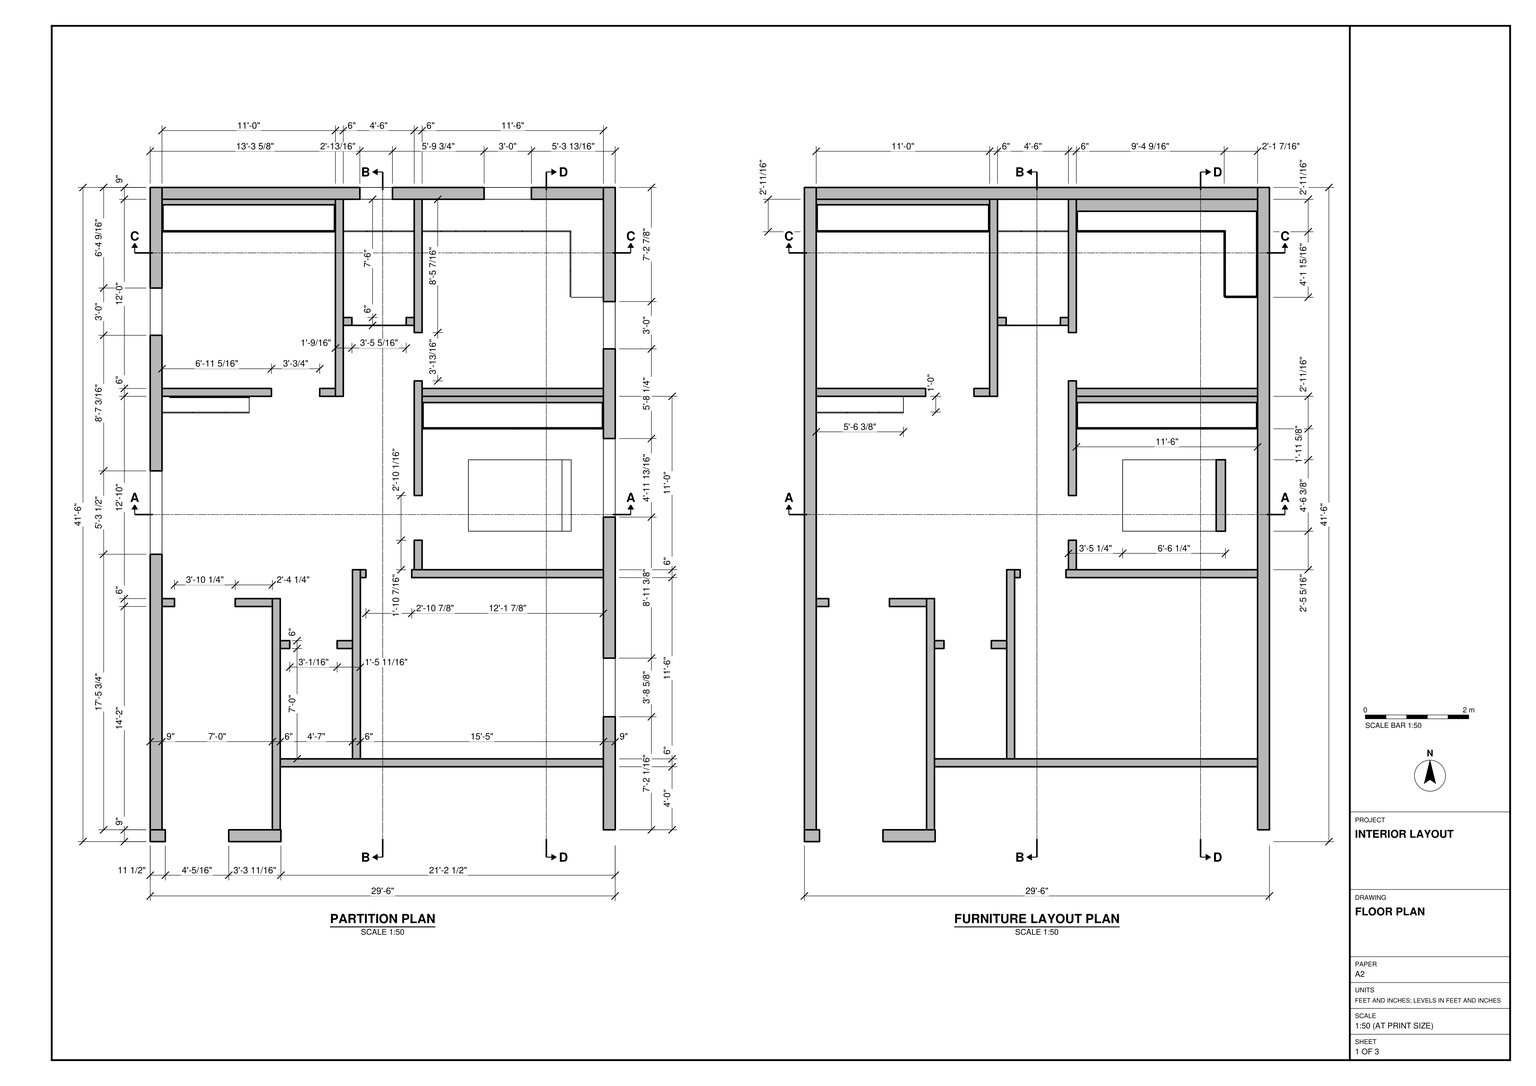
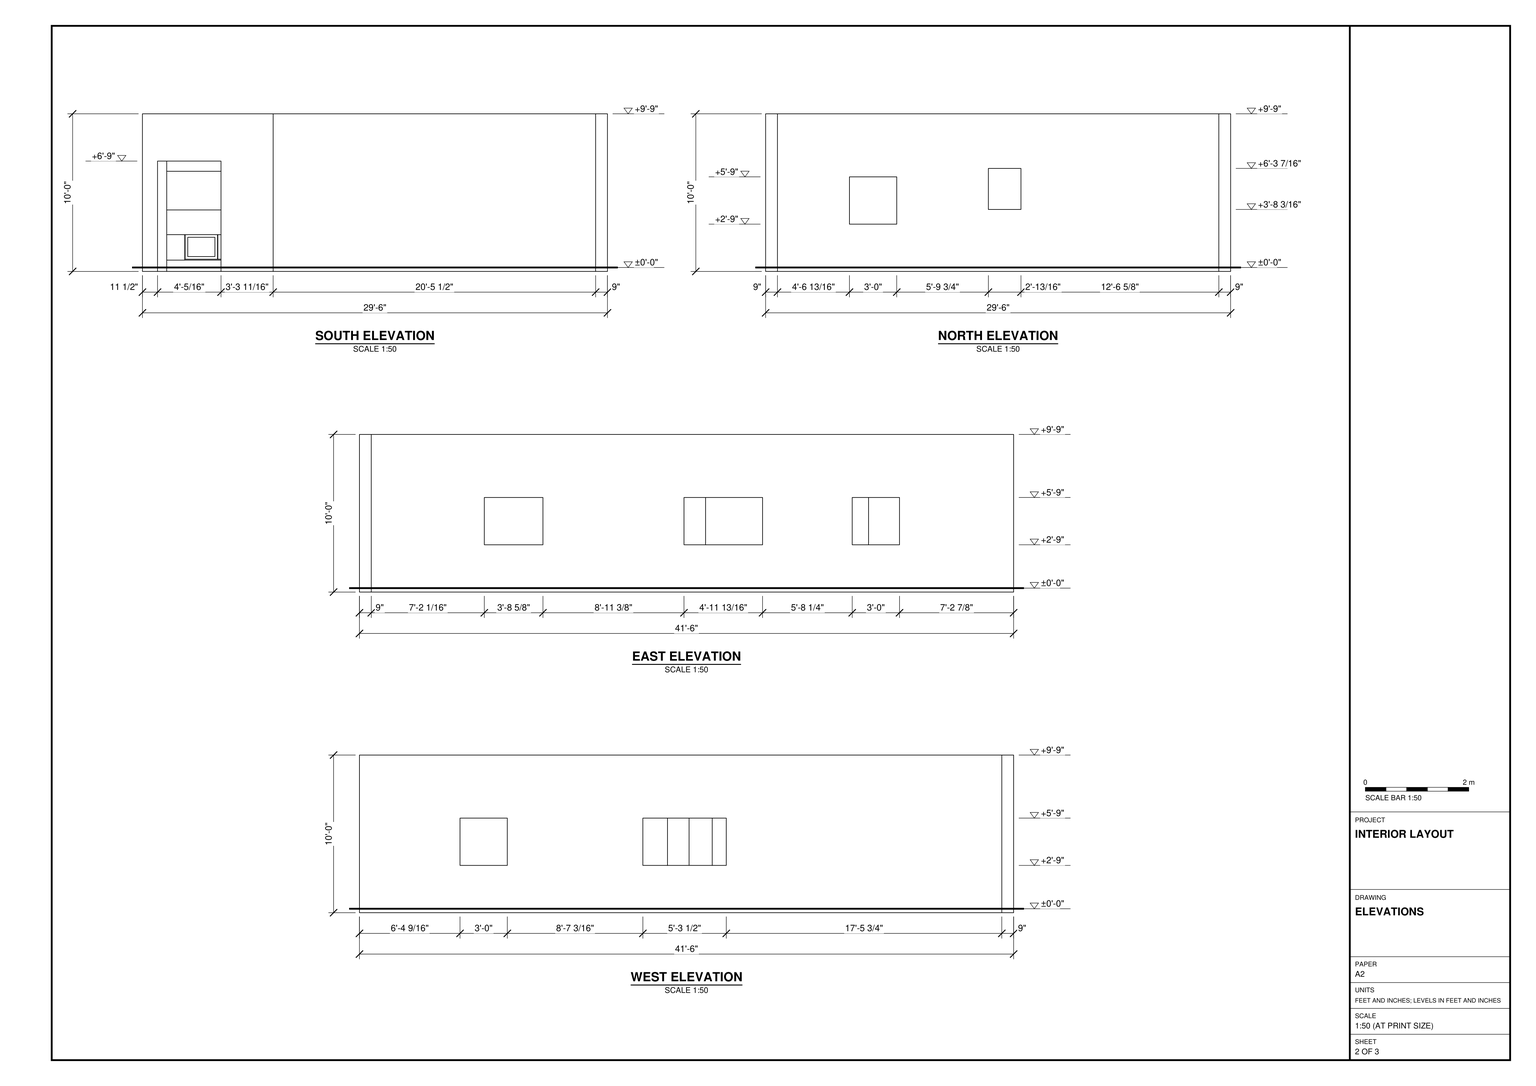
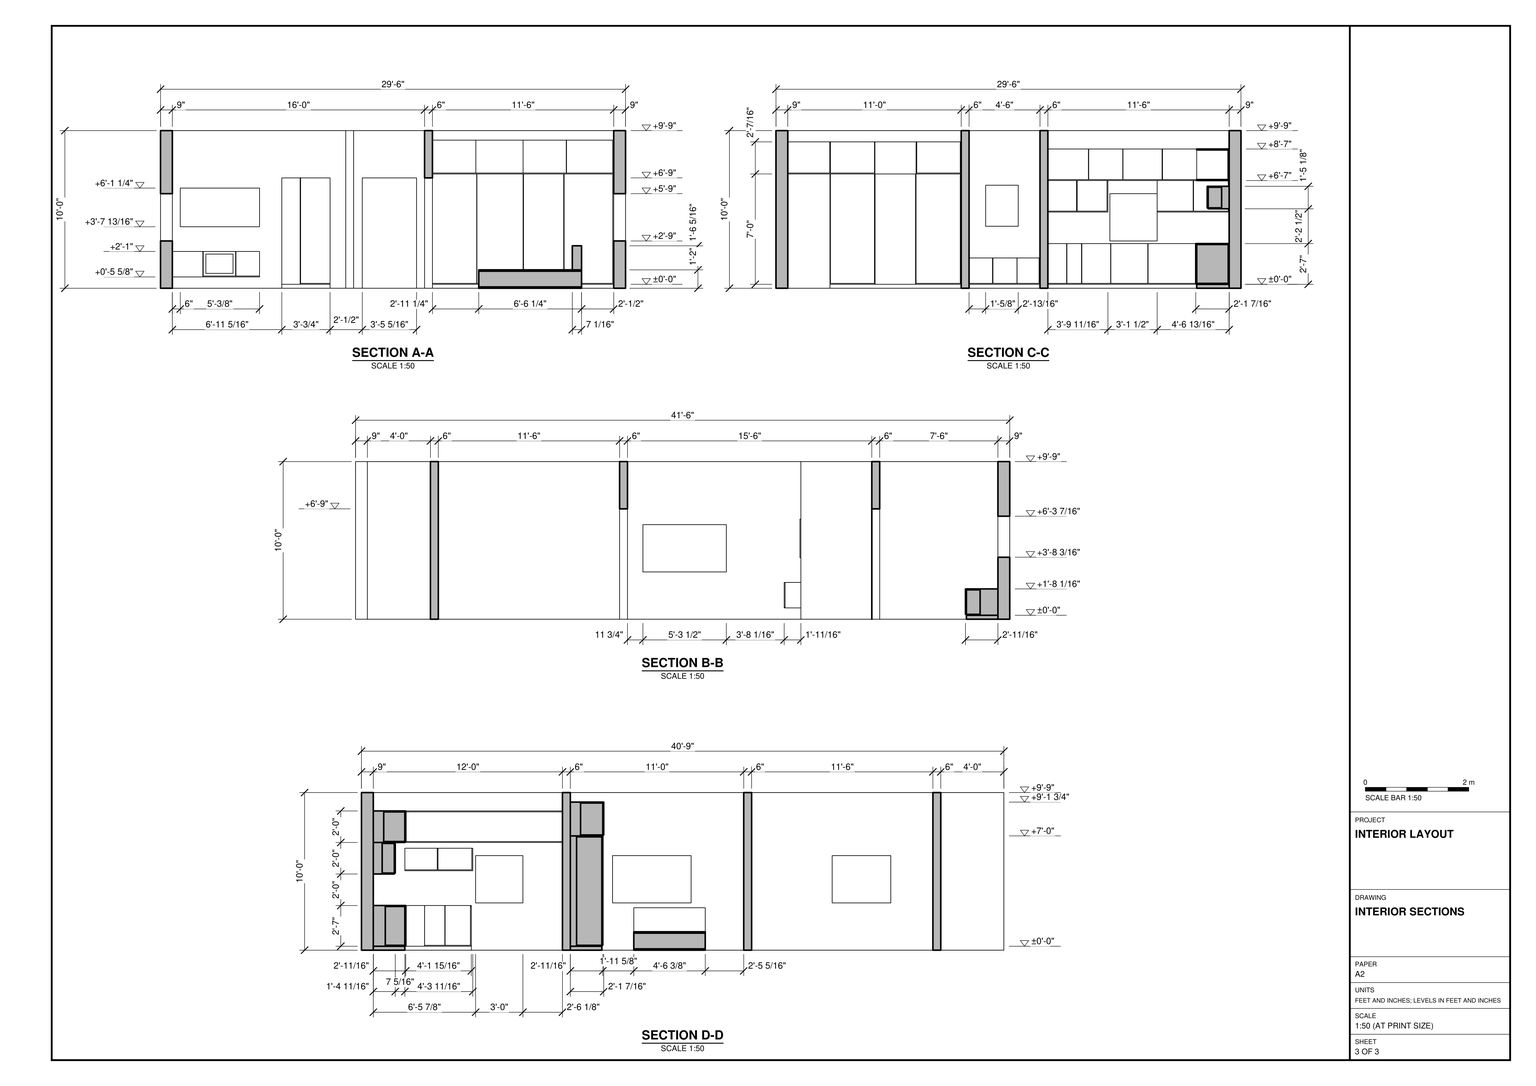
Build the interior in SketchUp from task_files/diagram_01.pdf. Work in feet and inches. Set the ground floor at ±0'-0" and make the model 29'-6" wide east to west, 41'-6" long north to south and 10'-0" high overall. The wall tops are at +9'-9" relative to the floor.

Use the partition plan to lay out the 9" perimeter walls and 6" internal partitions. Follow the setback at the south end, the narrow southwest entrance bay, the passages between rooms and the narrow bay between the two north rooms. Use the elevations to set the widths, sills and heads of the exterior openings; the two north windows have different sill heights.

Use the furniture plan for footprints and the interior sections for heights and cabinet divisions. Model the northwest storage run, the northeast kitchen cabinetry and its return, and the low wall unit on the passage side of the northwest room. Place the platform bed in the middle east room with its raised end to the east and the storage run along the north partition. Any decor or loose items shown may be represented by suitable library components.

Keep shell elements separate as groups or components, group each furniture or joinery piece separately, and use components for repeated parts. Save one SketchUp model as output_files/interior_with_fitted_cabinetry_and_platform_bed.skp.

# SketchUp Ruby script. Lengths in inches.
U = 1.inch
M = Sketchup.active_model
def pt(a) = Geom::Point3d.new(a.map { |v| v * U })
def face(e, loops, mat)
  f = e.add_face(loops[0].map { |a| pt(a) })
  loops[1..].each { |l| e.add_face(l.map { |a| pt(a) }).erase! }
  f.material = f.back_material = mat if mat
  f
end
# faces: each face lists its corners as indices into pts; further lists are holes
def faces(e, pts, list, mat = nil) = list.each { |f| face(e, (f[0].is_a?(Array) ? f : [f]).map { |l| l.map { |i| pts[i] } }, mat) }
# xy, xz, yz: faces in a plane at the given z, y or x. An outline is a flat list of corners, or four numbers for a rectangle; further outlines are holes
def ring(l) = l.size == 4 ? [[l[0], l[1]], [l[2], l[1]], [l[2], l[3]], [l[0], l[3]]] : l.each_slice(2).to_a
def flat(e, list, mat, &to3) = list.each { |f| face(e, (f[0].is_a?(Array) ? f : [f]).map { |l| ring(l).map { |u, v| to3.(u, v) } }, mat) }
def xy(e, z, list, mat = nil) = flat(e, list, mat) { |x, y| [x, y, z] }
def xz(e, y, list, mat = nil) = flat(e, list, mat) { |x, z| [x, y, z] }
def yz(e, x, list, mat = nil) = flat(e, list, mat) { |y, z| [x, y, z] }
def lines(e, pts, list) = list.each { |a, b| e.add_line(pt(pts[a]), pt(pts[b])) }
# prism: a flat outline (further loops are holes) pulled along v
def prism(e, loops, v, mat = nil)
  f = face(e, loops, mat); d = Geom::Vector3d.new(v.map { |x| x * U })
  f.pushpull(f.normal.samedirection?(d) ? d.length : -d.length)
end
def box(e, o, s, mat = nil) = prism(e, [[o, [o[0] + s[0], o[1], o[2]], [o[0] + s[0], o[1] + s[1], o[2]], [o[0], o[1] + s[1], o[2]]]], [0, 0, s[2]], mat)
def at(x, y, z, deg = 0) = Geom::Transformation.translation(pt([x, y, z])) * Geom::Transformation.rotation(ORIGIN, Z_AXIS, deg.degrees)
def axes(o, x, y, z) = Geom::Transformation.new([*x, 0, *y, 0, *z, 0, *pt(o).to_a, 1])
def part(name) = M.definitions.add(name)
# library, detail: a bought-in or finely detailed component or shape, given as its bounding box
def library(name, o, s) = part(name).tap { |d| box(d.entities, o, s) }
def detail(e, o, s) = box(e.add_group.entities, o, s)
def put(e, d, t, mat = nil) = e.add_instance(d, t).tap { |i| i.material = mat if mat }
def group(e, t, mat = nil) = e.add_group.tap { |g| g.transformation = t; g.material = mat if mat }.entities
root = M.entities
M.materials.add("[Translucent Glass Safety]").color = [204, 235, 244]
M.materials["[Translucent Glass Safety]"].alpha = 0.5
xz(root,393,[[153.57,0,194.89,84]],"[Translucent Glass Safety]")
g1 = group(root,at(0,0,0))
prism(g1,[[[99.51,9,0],[59.8125,9,0],[59.8125,9,84],[11.5,9,84],[11.5,9,0],[0,9,0],[0,9,120],[99.51,9,120]]],[0,-9,0])
g2 = group(root,at(0,9,0))
prism(g2,[[[0,489,0],[0,0,0],[0,0,120],[0,489,120]],[[0,273.25,72],[0,209.75,72],[0,209.75,36],[0,273.25,36]],[[0,412.4375,72],[0,376.4375,72],[0,376.4375,36],[0,412.4375,36]]],[9,0,0])
g3 = group(root,at(9,489,0))
prism(g3,[[[336,9,0],[0,9,0],[0,9,120],[336,9,120]],[[245.1875,9,36],[281.1875,9,36],[281.1875,9,72],[245.1875,9,72]],[[150.625,9,47.1875],[175.4375,9,47.1875],[175.4375,9,78.4375],[150.625,9,78.4375]]],[0,-9,0])
g4 = group(root,at(345,9,0))
prism(g4,[[[9,0,0],[9,489,0],[9,489,120],[9,0,120]],[[9,297.875,36],[9,238.0625,36],[9,238.0625,72],[9,297.875,72]],[[9,130.6875,36],[9,86.0625,36],[9,86.0625,72],[9,130.6875,72]],[[9,366.125,36],[9,366.125,72],[9,402.125,72],[9,402.125,36]]],[-9,0,0])
g5 = group(root,at(9,179,0))
prism(g5,[[[9.5,6,0],[0,6,0],[0,6,120],[84,6,120],[84,6,0],[55.73,6,0],[55.73,6,84],[9.5,6,84]]],[0,-6,0])
g6 = group(root,at(93,9,0))
box(g6,[0,0,0],[6,176,120])
g7 = group(root,at(99,57,0))
box(g7,[0,0,0],[246,6,120])
g8 = group(root,at(154,63,0))
box(g8,[0,0,0],[6,144,120])
g9 = group(root,at(99,147,0))
prism(g9,[[[55,6,0],[43.3125,6,0],[43.3125,6,84],[7.25,6,84],[7.25,6,0],[0,6,0],[0,6,120],[55,6,120]]],[0,-6,0])
g10 = group(root,at(160,201,0))
prism(g10,[[[4.25,6,0],[0,6,0],[0,6,120],[185,6,120],[185,6,0],[39.125,6,0],[39.125,6,84],[4.25,6,84]]],[0,-6,0])
g11 = group(root,at(141,339,0))
prism(g11,[[[6,0,0],[0,0,0],[0,6,0],[0,150,0],[6,150,0]]],[0,0,120])
g12 = group(root,at(9,339,0))
prism(g12,[[[0,0,0],[83.3125,0,0],[83.3125,0,84],[120.0625,0,84],[120.0625,0,0],[132,0,0],[132,0,120],[0,0,120]]],[0,6,0])
g13 = group(root,at(147,393,0))
prism(g13,[[[6.57,6,0],[0,6,0],[0,6,120],[54,6,120],[54,6,0],[47.89,6,0],[47.89,6,84],[6.57,6,84]]],[0,-6,0])
g14 = group(root,at(201,207,0))
prism(g14,[[[0,282,0],[0,180.5625,0],[0,180.5625,84],[0,143.75,84],[0,143.75,0],[0,56.5,0],[0,56.5,84],[0,22.4375,84],[0,22.4375,0],[0,0,0],[0,0,120],[0,282,120]]],[6,0,0])
g15 = group(root,at(207,339,0))
box(g15,[0,0,0],[138,6,120])
g16 = group(root,at(207,465,0))
prism(g16,[[[0,0,0],[0,24,0],[138,24,0],[138,-50.625,0],[113.29,-50.625,0],[113.29,0,0]]],[0,0,3])
g17 = group(root,at(207,465,3))
xy(g17,0,[[113.29,-50.625,113.29,0,0,0,0,24,138,24,138,-50.625]])
xy(g17,0.71,[[113.29,-50.625,137.29,-50.625,137.29,14.875,0.71,14.875,0.71,0,113.29,0]])
xy(g17,30.29,[[113.29,-50.625,113.29,0,0.71,0,0.71,14.875,137.29,14.875,137.29,-50.625]])
xy(g17,31,[[113.29,-50.625,138,-50.625,138,24,0,24,0,0,113.29,0]])
xz(g17,-50.625,[[113.29,0,138,0,138,31,113.29,31,113.29,30.29,137.29,30.29,137.29,0.71,113.29,0.71]])
xz(g17,0,[[0,0,113.29,0,113.29,0.71,0.71,0.71,0.71,30.29,113.29,30.29,113.29,31,0,31]])
xz(g17,14.875,[[0.71,0.71,137.29,30.29]])
xz(g17,24,[[0,0,138,31]])
yz(g17,0,[[0,0,24,31]])
yz(g17,0.71,[[0,0.71,14.875,30.29]])
yz(g17,113.29,[[-50.625,0,0,0.71],[-50.625,30.29,0,31]])
yz(g17,137.29,[[-50.625,0.71,14.875,30.29]])
yz(g17,138,[[-50.625,0,24,31]])
g18 = group(root,at(320.29,414.375,3.71))
box(g18,[0,0,0],[24,0.71,29.58])
g19 = group(root,at(207,464.29,3.71))
box(g19,[0,0,0],[14.27,0.71,30.29])
g20 = group(root,at(221.48,464.29,3.71))
box(g20,[0,0,0],[11.13,0.71,30.29])
g21 = group(root,at(232.86,464.29,3.71))
box(g21,[0,0,0],[21.9,0.71,30.29])
g22 = group(root,at(254.93,464.29,3.71))
box(g22,[0,0,0],[28.12,0.71,30.29])
g23 = group(root,at(283.27,464.29,3.71))
box(g23,[0,0,0],[37.02,0.71,30.29])
g24 = group(root,at(319.58,449.99,3))
box(g24,[0,0,0],[0.71,13.97,31])
g25 = group(root,at(319.58,434.56,3.71))
box(g25,[0,0,0],[0.71,15.375,30.29])
g26 = group(root,at(319.58,415.08,3.71))
box(g26,[0,0,0],[0.71,19.26,30.29])
g27 = group(root,at(207,489,58))
xy(g27,0,[[0,-16,45.6875,0]])
xy(g27,0.71,[[0.71,-16,44.98,-5.75]])
xy(g27,23.29,[[0.71,-16,44.98,-5.75]])
xy(g27,24,[[0,-16,45.6875,0]])
xz(g27,-16,[[[0,0,45.6875,24],[0.71,0.71,44.98,23.29]]])
xz(g27,-5.75,[[0.71,0.71,44.98,23.29]])
xz(g27,0,[[0,0,45.6875,24]])
yz(g27,0,[[-16,0,0,24]])
yz(g27,0.71,[[-16,0.71,-5.75,23.29]])
yz(g27,44.98,[[-16,0.71,-5.75,23.29]])
yz(g27,45.6875,[[-16,0,0,24]])
g28 = group(root,at(207,472.29,58.71))
box(g28,[0,0,0],[21.81,0.71,23.29])
g29 = group(root,at(229.3125,472.29,58.71))
box(g29,[0,0,0],[22.66,0.71,23.29])
g30 = group(root,at(290.1875,489,58))
xy(g30,0,[[0,-16,54.8125,0]])
xy(g30,0.71,[[0.71,-16,54.1,-6.75]])
xy(g30,23.29,[[0.71,-16,54.1,-6.75]])
xy(g30,24,[[0,-16,54.8125,0]])
xz(g30,-16,[[[0,0,54.8125,24],[0.71,0.71,54.1,23.29]]])
xz(g30,-6.75,[[0.71,0.71,54.1,23.29]])
xz(g30,0,[[0,0,54.8125,24]])
yz(g30,0,[[-16,0,0,24]])
yz(g30,0.71,[[-16,0.71,-6.75,23.29]])
yz(g30,54.1,[[-16,0.71,-6.75,23.29]])
yz(g30,54.8125,[[-16,0,0,24]])
g31 = group(root,at(290.1875,472.29,58.71))
box(g31,[0,0,0],[27.41,0.71,23.29])
g32 = group(root,at(317.89,472.29,58.71))
box(g32,[0,0,0],[26.4,0.71,23.29])
g33 = group(root,at(345,413.29,60.48))
xy(g33,0,[[-16,0,0,51.6875]])
xy(g33,0.71,[[-16,0.71,-5.75,50.98]])
xy(g33,16.42,[[-16,0.71,-5.75,50.98]])
xy(g33,17.125,[[-16,0,0,51.6875]])
xz(g33,0,[[-16,0,0,17.125]])
xz(g33,0.71,[[-16,0.71,-5.75,16.42]])
xz(g33,50.98,[[-16,0.71,-5.75,16.42]])
xz(g33,51.6875,[[-16,0,0,17.125]])
yz(g33,-16,[[[0,0,51.6875,17.125],[0.71,0.71,50.98,16.42]]])
yz(g33,-5.75,[[0.71,0.71,50.98,16.42]])
yz(g33,0,[[0,0,51.6875,17.125]])
g34 = group(root,at(328.29,440.33,61.19))
box(g34,[0,0,0],[0.71,24.64,16.42])
g35 = group(root,at(328.29,413.99,61.19))
box(g35,[0,0,0],[0.71,25.75,16.42])
g36 = group(root,at(207,489,82))
xy(g36,0,[[113.29,-144,113.29,-24,0,-24,0,0,138,0,138,-144]])
xy(g36,0.71,[[113.29,-144,137.29,-144,137.29,-7.9375,0.71,-7.9375,0.71,-24,113.29,-24]])
xy(g36,23.29,[[113.29,-144,113.29,-24,0.71,-24,0.71,-7.9375,137.29,-7.9375,137.29,-144]])
xy(g36,24,[[113.29,-144,138,-144,138,0,0,0,0,-24,113.29,-24]])
xz(g36,-144,[[113.29,0,138,0,138,24,113.29,24,113.29,23.29,137.29,23.29,137.29,0.71,113.29,0.71]])
xz(g36,-24,[[0,0,113.29,0,113.29,0.71,0.71,0.71,0.71,23.29,113.29,23.29,113.29,24,0,24]])
xz(g36,-7.9375,[[0.71,0.71,137.29,23.29]])
xz(g36,0,[[0,0,138,24]])
yz(g36,0,[[-24,0,0,24]])
yz(g36,0.71,[[-24,0.71,-7.9375,23.29]])
yz(g36,113.29,[[-144,0,-24,0.71],[-144,23.29,-24,24]])
yz(g36,137.29,[[-144,0.71,-7.9375,23.29]])
yz(g36,138,[[-144,0,0,24]])
g37 = group(root,at(207,464.29,82.71))
box(g37,[0,0,0],[30.84,0.71,23.29])
g38 = group(root,at(238.09,464.29,82.71))
box(g38,[0,0,0],[25.91,0.71,23.29])
g39 = group(root,at(264.19,464.29,82.71))
box(g39,[0,0,0],[29.72,0.71,23.29])
g40 = group(root,at(294.27,464.29,82.71))
box(g40,[0,0,0],[26.02,0.71,23.29])
g41 = group(root,at(9,465,0))
box(g41,[0,0,0],[132,24,3])
g42 = group(root,at(9,465,3))
xy(g42,0,[[0,0,132,24]])
xy(g42,0.71,[[0.71,0,131.29,19.8125]])
xy(g42,83.29,[[0.71,0,131.29,19.8125]])
xy(g42,84,[[0,0,132,24]])
xz(g42,0,[[[0,0,132,84],[0.71,0.71,131.29,83.29]]])
xz(g42,19.8125,[[0.71,0.71,131.29,83.29]])
xz(g42,24,[[0,0,132,84]])
yz(g42,0,[[0,0,24,84]])
yz(g42,0.71,[[0,0.71,19.8125,83.29]])
yz(g42,131.29,[[0,0.71,19.8125,83.29]])
yz(g42,132,[[0,0,24,84]])
g43 = group(root,at(9,464.29,0))
box(g43,[0,0,0],[32.11,0.71,87])
g44 = group(root,at(41.47,464.29,3.71))
box(g44,[0,0,0],[33.53,0.71,83.29])
g45 = group(root,at(75.46,464.29,3))
box(g45,[0,0,0],[30.81,0.71,84])
g46 = group(root,at(106.65,464.29,3.71))
box(g46,[0,0,0],[33.64,0.71,83.29])
g47 = group(root,at(9,489,87))
xy(g47,0,[[0,-24.71,132,0]])
xy(g47,0.71,[[0.71,-24.71,131.29,-8.15]])
xy(g47,23.74,[[0.71,-24.71,131.29,-8.15]])
xy(g47,24.45,[[0,-24.71,132,0]])
xz(g47,-24.71,[[[0,0,132,24.45],[0.71,0.71,131.29,23.74]]])
xz(g47,-8.15,[[0.71,0.71,131.29,23.74]])
xz(g47,0,[[0,0,132,24.45]])
yz(g47,0,[[-24.71,0,0,24.45]])
yz(g47,0.71,[[-24.71,0.71,-8.15,23.74]])
yz(g47,131.29,[[-24.71,0.71,-8.15,23.74]])
yz(g47,132,[[-24.71,0,0,24.45]])
g48 = group(root,at(9,463.58,87.71))
box(g48,[0,0,0],[31.97,0.71,23.74])
g49 = group(root,at(41.47,463.58,87.71))
box(g49,[0,0,0],[33.53,0.71,23.74])
g50 = group(root,at(75.34,463.58,87))
box(g50,[0,0,0],[31.31,0.71,24.45])
g51 = group(root,at(107.2,463.58,87.71))
box(g51,[0,0,0],[33.09,0.71,23.74])
g52 = group(root,at(147,465,0))
box(g52,[0,0,0],[54,24,3])
g53 = group(root,at(147,465,3))
xy(g53,0,[[0,0,54,24]])
xy(g53,0.71,[[0.71,0,53.29,10.4375]])
xy(g53,19.35,[[0.71,0,53.29,10.4375]])
xy(g53,20.0625,[[0,0,54,24]])
xz(g53,0,[[[0,0,54,20.0625],[0.71,0.71,53.29,19.35]]])
xz(g53,10.4375,[[0.71,0.71,53.29,19.35]])
xz(g53,24,[[0,0,54,20.0625]])
yz(g53,0,[[0,0,24,20.0625]])
yz(g53,0.71,[[0,0.71,10.4375,19.35]])
yz(g53,53.29,[[0,0.71,10.4375,19.35]])
yz(g53,54,[[0,0,24,20.0625]])
g54 = group(root,at(147,464.29,3.71))
box(g54,[0,0,0],[17.87,0.71,19.35])
g55 = group(root,at(165.1875,464.29,3.71))
box(g55,[0,0,0],[18.28,0.71,19.35])
g56 = group(root,at(183.55,464.29,3.71))
box(g56,[0,0,0],[16.74,0.71,19.35])
g57 = group(root,at(207,315,0))
box(g57,[0,0,0],[138,24,3])
g58 = group(root,at(207,315,3))
xy(g58,0,[[0,0,138,24]])
xy(g58,0.71,[[0.71,0,137.29,19.25]])
xy(g58,83.29,[[0.71,0,137.29,19.25]])
xy(g58,84,[[0,0,138,24]])
xz(g58,0,[[[0,0,138,84],[0.71,0.71,137.29,83.29]]])
xz(g58,19.25,[[0.71,0.71,137.29,83.29]])
xz(g58,24,[[0,0,138,84]])
yz(g58,0,[[0,0,24,84]])
yz(g58,0.71,[[0,0.71,19.25,83.29]])
yz(g58,137.29,[[0,0.71,19.25,83.29]])
yz(g58,138,[[0,0,24,84]])
g59 = group(root,at(207,314.29,3.71))
box(g59,[0,0,0],[33.67,0.71,83.29])
g60 = group(root,at(240.86,314.29,3.71))
box(g60,[0,0,0],[35.14,0.71,83.29])
g61 = group(root,at(276.33,314.29,3.71))
box(g61,[0,0,0],[30.6,0.71,83.29])
g62 = group(root,at(307.25,314.29,3.71))
box(g62,[0,0,0],[37.05,0.71,83.29])
g63 = group(root,at(207,339,87))
xy(g63,0,[[0,-24.71,138,0]])
xy(g63,0.71,[[0.71,-24.71,137.29,-7.77]])
xy(g63,25.04,[[0.71,-24.71,137.29,-7.77]])
xy(g63,25.75,[[0,-24.71,138,0]])
xz(g63,-24.71,[[[0,0,138,25.75],[0.71,0.71,137.29,25.04]]])
xz(g63,-7.77,[[0.71,0.71,137.29,25.04]])
xz(g63,0,[[0,0,138,25.75]])
yz(g63,0,[[-24.71,0,0,25.75]])
yz(g63,0.71,[[-24.71,0.71,-7.77,25.04]])
yz(g63,137.29,[[-24.71,0.71,-7.77,25.04]])
yz(g63,138,[[-24.71,0,0,25.75]])
g64 = group(root,at(207,313.58,87.71))
box(g64,[0,0,0],[33.04,0.71,25.04])
g65 = group(root,at(240.04,313.58,87.71))
box(g65,[0,0,0],[35.96,0.71,25.04])
g66 = group(root,at(276,313.58,87.71))
box(g66,[0,0,0],[32.85,0.71,25.04])
g67 = group(root,at(309.07,313.58,87.71))
box(g67,[0,0,0],[35.22,0.71,25.04])
g68 = group(root,at(242.26,236.3125,0))
box(g68,[0,0,0],[78.25,54.375,1])
g69 = group(root,at(242.26,236.3125,1))
box(g69,[0,0,0],[78.25,54.375,12])
g70 = group(root,at(242.26,236.3125,13))
box(g70,[0,0,0],[78.25,54.375,1])
g71 = group(root,at(313.46,236.3125,14))
box(g71,[0,0,0],[7.04,54.375,18.3125])
g72 = group(root,at(9,339,8.61))
xy(g72,0,[[0,-12,66.375,0]])
xy(g72,0.71,[[0.71,-12,65.67,-4]])
xy(g72,18.68,[[0.71,-12,65.67,-4]])
xy(g72,19.39,[[0,-12,66.375,0]])
xz(g72,-12,[[[0,0,66.375,19.39],[0.71,0.71,65.67,18.68]]])
xz(g72,-4,[[0.71,0.71,65.67,18.68]])
xz(g72,0,[[0,0,66.375,19.39]])
yz(g72,0,[[-12,0,0,19.39]])
yz(g72,0.71,[[-12,0.71,-4,18.68]])
yz(g72,65.67,[[-12,0.71,-4,18.68]])
yz(g72,66.375,[[-12,0,0,19.39]])
g73 = group(root,at(9,326.29,8.61))
box(g73,[0,0,0],[23.22,0.71,19.39])
g74 = group(root,at(32.51,326.29,9.32))
prism(g74,[[[24.67,0,0],[24.67,0,18.68],[0,0,18.68],[0,0,0]],[[2,0,2],[2,0,16.68],[22.67,0,16.68],[22.67,0,2]]],[0,0.71,0])
g75 = group(root,at(57.42,326.29,9.32))
box(g75,[0,0,0],[17.96,0.71,18.68])
g76 = group(root,at(15.03,339,46.8125))
box(g76,[0,-0.71,0],[60.35,0.71,29.4375])
